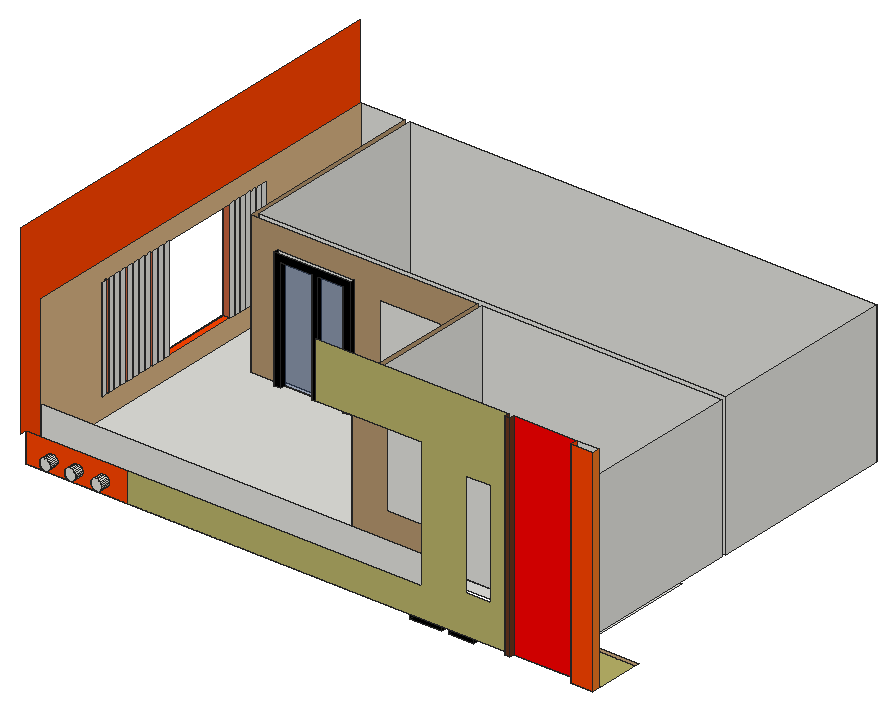
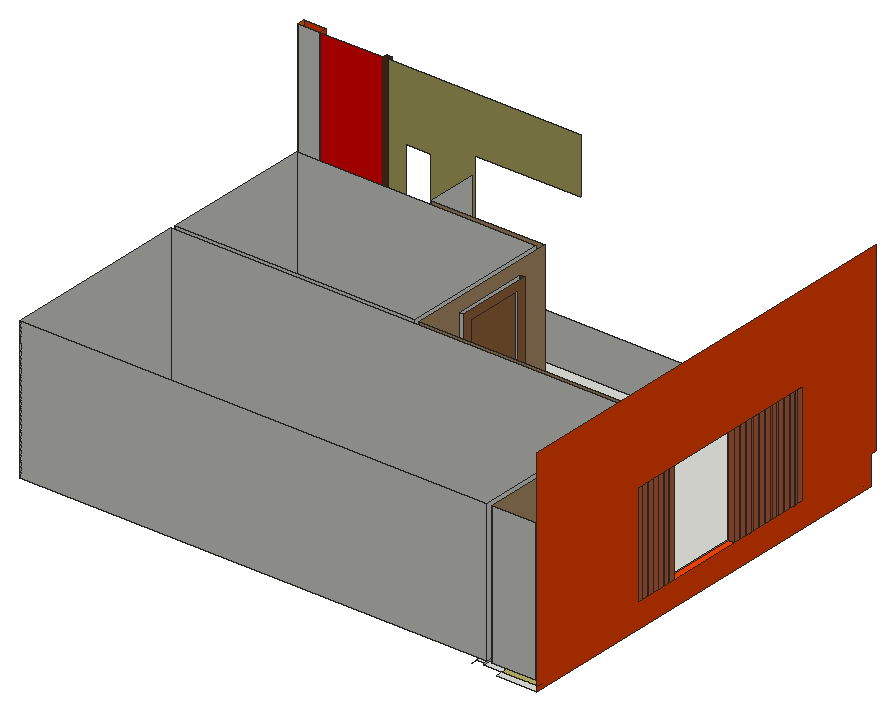
# SketchUp Ruby script. Lengths in inches.
U = 1.inch
M = Sketchup.active_model
def pt(a) = Geom::Point3d.new(a.map { |v| v * U })
def face(e, loops, mat)
  f = e.add_face(loops[0].map { |a| pt(a) })
  loops[1..].each { |l| e.add_face(l.map { |a| pt(a) }).erase! }
  f.material = f.back_material = mat if mat
  f
end
# faces: each face lists its corners as indices into pts; further lists are holes
def faces(e, pts, list, mat = nil) = list.each { |f| face(e, (f[0].is_a?(Array) ? f : [f]).map { |l| l.map { |i| pts[i] } }, mat) }
# xy, xz, yz: faces in a plane at the given z, y or x. An outline is a flat list of corners, or four numbers for a rectangle; further outlines are holes
def ring(l) = l.size == 4 ? [[l[0], l[1]], [l[2], l[1]], [l[2], l[3]], [l[0], l[3]]] : l.each_slice(2).to_a
def flat(e, list, mat, &to3) = list.each { |f| face(e, (f[0].is_a?(Array) ? f : [f]).map { |l| ring(l).map { |u, v| to3.(u, v) } }, mat) }
def xy(e, z, list, mat = nil) = flat(e, list, mat) { |x, y| [x, y, z] }
def xz(e, y, list, mat = nil) = flat(e, list, mat) { |x, z| [x, y, z] }
def yz(e, x, list, mat = nil) = flat(e, list, mat) { |y, z| [x, y, z] }
def lines(e, pts, list) = list.each { |a, b| e.add_line(pt(pts[a]), pt(pts[b])) }
# prism: a flat outline (further loops are holes) pulled along v
def prism(e, loops, v, mat = nil)
  f = face(e, loops, mat); d = Geom::Vector3d.new(v.map { |x| x * U })
  f.pushpull(f.normal.samedirection?(d) ? d.length : -d.length)
end
def box(e, o, s, mat = nil) = prism(e, [[o, [o[0] + s[0], o[1], o[2]], [o[0] + s[0], o[1] + s[1], o[2]], [o[0], o[1] + s[1], o[2]]]], [0, 0, s[2]], mat)
def at(x, y, z, deg = 0) = Geom::Transformation.translation(pt([x, y, z])) * Geom::Transformation.rotation(ORIGIN, Z_AXIS, deg.degrees)
def axes(o, x, y, z) = Geom::Transformation.new([*x, 0, *y, 0, *z, 0, *pt(o).to_a, 1])
def part(name) = M.definitions.add(name)
# library, detail: a bought-in or finely detailed component or shape, given as its bounding box
def library(name, o, s) = part(name).tap { |d| box(d.entities, o, s) }
def detail(e, o, s) = box(e.add_group.entities, o, s)
def put(e, d, t, mat = nil) = e.add_instance(d, t).tap { |i| i.material = mat if mat }
def group(e, t, mat = nil) = e.add_group.tap { |g| g.transformation = t; g.material = mat if mat }.entities
root = M.entities
M.materials.add("[0020_Red]").color = [255, 0, 0]
M.materials.add("[0024_OrangeRed]").color = [255, 69, 0]
M.materials.add("[0025_Coral]").color = [198, 99, 62]
M.materials.add("[0036_BurlyWood]").color = [181, 150, 110]
M.materials.add("[0036_BurlyWood]4").color = [216, 179, 131]
M.materials.add("[0041_Chocolate]1").color = [239, 119, 34]
M.materials.add("[0042_Sienna]").color = [104, 53, 29]
M.materials.add("[0057_DarkKhaki]").color = [186, 180, 105]
M.materials.add("[0137_Black]").color = [0, 0, 0]
M.materials.add("[Color M09]").color = [0, 0, 0]
M.materials.add("[Translucent Glass Blue]").color = [51, 76, 122]
M.materials["[Translucent Glass Blue]"].alpha = 0.5
M.materials.add("[Translucent Glass Gray]").color = [165, 165, 165]
M.materials["[Translucent Glass Gray]"].alpha = 0.5
M.materials.add("[Wood Bamboo]").color = [196, 88, 55]
M.materials.add("[Wood Floor Parquet]").color = [145, 89, 39]
M.materials.add("[Wood Floor]").color = [155, 105, 61]
xy(root,130.33,[[443.09,303.3125,483.76,309.3125],[492.14,303.3125,524.43,309.3125]],"[0137_Black]")
xy(root,132.36,[[129.72,453.875,217.79,454.875]],"[Wood Bamboo]")
xy(root,138.4375,[[379.5,353.72,382.5,429.09]],"[Wood Floor Parquet]")
xy(root,140.42,[[254.5625,454.875,298.59,457.875],[303.24,454.875,342.625,457.875]],"[0137_Black]")
xy(root,144.3,[[379.5,347.86,385.5,434.95]],"[Wood Floor Parquet]")
xy(root,144.99,[[443.09,303.3125,483.76,309.3125],[492.14,303.3125,524.43,309.3125]],"[0137_Black]")
xy(root,147.14,[[247.84,454.875,349.34,457.875]])
xy(root,153.6875,[[129.72,451.875,217.79,454.875]],"[Wood Bamboo]")
xy(root,155.1,[[432.98,303.3125,534.54,309.3125]],"[0137_Black]")
xy(root,159.6875,[[123.72,451.875,223.79,457.875]],"[Wood Bamboo]")
xy(root,177.375,[[51.5625,457.875,74.75,463.875],[51.5625,463.875,74.75,767.8125],[0,767.8125,51.5625,776.8125]])
xy(root,177.375,[[537.22,303.3125,730.1875,309.3125]],"[0036_BurlyWood]")
xy(root,177.375,[[701.81,236.125,730.1875,245.125]],"[0041_Chocolate]1")
xy(root,177.375,[[615.29,239.125,615.29,245.125,0,245.125,0,248.25,730.1875,248.25,730.1875,245.125,621.57,245.125,621.57,239.125],[0,248.25,0,767.8125,51.5625,767.8125,51.5625,457.875,385.5,457.875,385.5,309.3125,537.22,309.3125,537.22,303.3125,730.1875,303.3125,730.1875,248.25]],"[0057_DarkKhaki]")
xy(root,180,[[385.5,309.3125,391.5,315.3125],[391.5,315.3125,665.75,457.875],[74.75,457.875,83.75,463.875],[74.75,463.875,83.75,767.8125]])
xy(root,183,[[9,257.25,498.8125,257.25,498.8125,321.9375,354.4375,321.9375,354.4375,361.01,348.4375,361.01,348.4375,372.41,351.4375,372.41,351.4375,446.78,348.4375,446.78,348.4375,458.18,354.4375,458.18,354.4375,521.4375,197.41,521.4375,197.41,515.4375,188.31,515.4375,188.31,521.4375,155.35,521.4375,155.35,515.4375,148.77,515.4375,148.77,521.4375,109.24,521.4375,109.24,515.4375,100.13,515.4375,100.13,521.4375,65.25,521.4375,65.25,767.8125,9,767.8125],[360.4375,327.9375,665.75,521.4375],[348.4375,361.01,354.4375,372.41],[351.4375,372.41,354.4375,446.78],[348.4375,446.78,354.4375,458.18],
  [100.13,515.4375,109.24,521.4375],[148.77,515.4375,155.35,521.4375],[188.31,515.4375,197.41,521.4375],[71.25,527.4375,665.75,767.8125]])
xy(root,208.56,[[0,355.7,9,361.9],[0,365.65,9,365.7],[0,365.7,9,371.9],[0,375.7,9,381.9],[0,385.7,9,391.9],
  [0,395.7,9,401.9],[0,405.7,9,411.9],[0,415.7,9,421.9],[0,425.7,9,431.9],[0,435.7,9,441.9],
  [0,445.7,9,451.9],[0,455.7,9,461.9],[0,559.26,9,565.46],[0,565.46,9,567.7],[0,567.7,9,573.9],
  [0,573.9,9,576.14],[0,576.14,9,582.34],[0,582.34,9,584.57],[0,584.57,9,590.78],[0,590.78,9,593.01],
  [0,593.01,9,599.21],[0,599.21,9,601.45],[0,601.45,9,607.65],[0,607.65,9,609.89],[0,609.89,9,616.09],
  [0,616.09,9,616.14]])
xy(root,208.56,[[0,461.9,9,559.26]],"[0024_OrangeRed]")
xy(root,208.56,[[0,352.64,9,355.7],[0,361.9,9,365.65],[0,371.9,9,375.7],[0,381.9,9,385.7],[0,391.9,9,395.7],
  [0,401.9,9,405.7],[0,411.9,9,415.7],[0,421.9,9,425.7],[0,431.9,9,435.7],[0,441.9,9,445.7],
  [0,451.9,9,455.7]],"[0025_Coral]")
xz(root,233.5625,[[33.6875,185.625,35.55,185.87,37.28,186.59,38.77,187.73,39.91,189.22,40.63,190.95,40.875,192.8125,40.63,194.67,39.91,196.41,38.77,197.9,37.28,199.04,35.55,199.76,33.6875,200,31.83,199.76,30.09,199.04,28.6,197.9,27.46,196.41,26.74,194.67,26.5,192.8125,26.74,190.95,27.46,189.22,28.6,187.73,30.09,186.59,31.83,185.87],[65.6875,185.625,67.55,185.87,69.28,186.59,70.77,187.73,71.91,189.22,72.63,190.95,72.875,192.8125,72.63,194.67,71.91,196.41,70.77,197.9,69.28,199.04,67.55,199.76,65.6875,200,63.83,199.76,62.09,199.04,60.6,197.9,59.46,196.41,58.74,194.67,58.5,192.8125,58.74,190.95,59.46,189.22,60.6,187.73,62.09,186.59,63.83,185.87],[99.0625,185.625,100.92,185.87,102.66,186.59,104.14,187.73,105.29,189.22,106,190.95,106.25,192.8125,106,194.67,105.29,196.41,104.14,197.9,102.66,199.04,100.92,199.76,99.0625,200,97.2,199.76,95.47,199.04,93.98,197.9,92.84,196.41,92.12,194.67,91.875,192.8125,92.12,190.95,92.84,189.22,93.98,187.73,95.47,186.59,97.2,185.87]])
xz(root,236.125,[[701.81,177.375,730.1875,450]],"[0024_OrangeRed]")
xz(root,239.125,[[615.29,177.375,621.57,450]],"[0042_Sienna]")
xz(root,245.125,[[701.81,177.375,730.1875,450]])
xz(root,245.125,[[621.57,177.375,701.81,450]],"[0020_Red]")
xz(root,245.125,[[[0,177.375,130.26,214.625],[99.0625,185.625,97.2,185.87,95.47,186.59,93.98,187.73,92.84,189.22,92.12,190.95,91.875,192.8125,92.12,194.67,92.84,196.41,93.98,197.9,95.47,199.04,97.2,199.76,99.0625,200,100.92,199.76,102.66,199.04,104.14,197.9,105.29,196.41,106,194.67,106.25,192.8125,106,190.95,105.29,189.22,104.14,187.73,102.66,186.59,100.92,185.87],[65.6875,185.625,63.83,185.87,62.09,186.59,60.6,187.73,59.46,189.22,58.74,190.95,58.5,192.8125,58.74,194.67,59.46,196.41,60.6,197.9,62.09,199.04,63.83,199.76,65.6875,200,67.55,199.76,69.28,199.04,70.77,197.9,71.91,196.41,72.63,194.67,72.875,192.8125,72.63,190.95,71.91,189.22,70.77,187.73,69.28,186.59,67.55,185.87],[33.6875,185.625,31.83,185.87,30.09,186.59,28.6,187.73,27.46,189.22,26.74,190.95,26.5,192.8125,26.74,194.67,27.46,196.41,28.6,197.9,30.09,199.04,31.83,199.76,33.6875,200,35.55,199.76,37.28,199.04,38.77,197.9,39.91,196.41,40.63,194.67,40.875,192.8125,40.63,190.95,39.91,189.22,38.77,187.73,37.28,186.59,35.55,185.87]]],"[0024_OrangeRed]")
xz(root,245.125,[[[130.26,177.375,615.29,177.375,615.29,450,369.99,450,369.99,378.625,504.125,378.625,504.125,214.625,130.26,214.625],[561.28,226.86,593.09,360.8]]],"[0057_DarkKhaki]")
xz(root,257.25,[[9,183,498.8125,243]])
xz(root,309.3125,[[385.5,177.375,391.5,180]])
xz(root,309.3125,[[443.09,130.33,483.76,144.99],[492.14,130.33,524.43,144.99]],"[Translucent Glass Gray]")
xz(root,321.9375,[[[354.4375,183,498.8125,363],[398.32,228.95,478.64,338.07]]],"[0036_BurlyWood]")
xz(root,327.9375,[[360.4375,183,665.75,363]])
xz(root,352.64,[[0,208.56,9,339.56]],"[0025_Coral]")
xz(root,355.7,[[0,208.56,9,339.56]],"[0025_Coral]")
xz(root,361.01,[[348.4375,183,354.4375,345.77]],"[Wood Floor]")
xz(root,361.9,[[0,208.56,9,339.56]],"[0025_Coral]")
xz(root,365.65,[[0,208.56,9,339.56]],"[0025_Coral]")
xz(root,371.9,[[0,208.56,9,339.56]],"[0025_Coral]")
xz(root,372.41,[[348.4375,183,351.4375,334.375]])
xz(root,375.7,[[0,208.56,9,339.56]],"[0025_Coral]")
xz(root,381.9,[[0,208.56,9,339.56]],"[0025_Coral]")
xz(root,385.7,[[0,208.56,9,339.56]],"[0025_Coral]")
xz(root,391.9,[[0,208.56,9,339.56]],"[0025_Coral]")
xz(root,395.7,[[0,208.56,9,339.56]],"[0025_Coral]")
xz(root,401.9,[[0,208.56,9,339.56]],"[0025_Coral]")
xz(root,405.7,[[0,208.56,9,339.56]],"[0025_Coral]")
xz(root,411.9,[[0,208.56,9,339.56]],"[0025_Coral]")
xz(root,415.7,[[0,208.56,9,339.56]],"[0025_Coral]")
xz(root,421.9,[[0,208.56,9,339.56]],"[0025_Coral]")
xz(root,425.7,[[0,208.56,9,339.56]],"[0025_Coral]")
xz(root,431.9,[[0,208.56,9,339.56]],"[0025_Coral]")
xz(root,435.7,[[0,208.56,9,339.56]],"[0025_Coral]")
xz(root,441.9,[[0,208.56,9,339.56]],"[0025_Coral]")
xz(root,445.7,[[0,208.56,9,339.56]],"[0025_Coral]")
xz(root,446.78,[[348.4375,183,351.4375,334.375]],"[Wood Floor]")
xz(root,451.9,[[0,208.56,9,339.56]],"[0025_Coral]")
xz(root,454.875,[[129.72,132.36,217.79,153.6875]],"[Wood Bamboo]")
xz(root,455.7,[[0,208.56,9,339.69]],"[0025_Coral]")
xz(root,457.875,[[74.75,177.375,83.75,180]])
xz(root,458.18,[[348.4375,183,354.4375,345.77]])
xz(root,461.9,[[0,208.56,9,339.69]],"[0025_Coral]")
xz(root,515.4375,[[100.13,183,109.24,183,109.24,326.0625,148.77,326.0625,148.77,183,155.35,183,155.35,326.0625,188.31,326.0625,188.31,183,197.41,183,197.41,335.17,100.13,335.17]],"[0137_Black]")
xz(root,521.4375,[[100.13,173.89,197.41,183],[360.4375,183,665.75,363]])
xz(root,521.4375,[[[65.25,183,100.13,183,100.13,335.17,197.41,335.17,197.41,183,354.4375,183,354.4375,363,65.25,363],[230.26,235.22,307.58,323.78]]],"[0036_BurlyWood]")
xz(root,521.4375,[[109.24,183,148.77,326.0625],[155.35,183,188.31,326.0625]],"[Translucent Glass Blue]")
xz(root,527.4375,[[71.25,183,665.75,363]])
xz(root,559.26,[[0,208.56,9,339.56]],"[0025_Coral]")
xz(root,565.46,[[0,208.56,9,339.56]],"[0025_Coral]")
xz(root,567.7,[[0,208.56,9,339.56]],"[0025_Coral]")
xz(root,573.9,[[0,208.56,9,339.56]],"[0025_Coral]")
xz(root,576.14,[[0,208.56,9,339.56]],"[0025_Coral]")
xz(root,582.34,[[0,208.56,9,339.56]],"[0025_Coral]")
xz(root,584.57,[[0,208.56,9,339.56]],"[0025_Coral]")
xz(root,590.78,[[0,208.56,9,339.56]],"[0025_Coral]")
xz(root,593.01,[[0,208.56,9,339.56]],"[0025_Coral]")
xz(root,599.21,[[0,208.56,9,339.56]],"[0025_Coral]")
xz(root,601.45,[[0,208.56,9,339.56]],"[0025_Coral]")
xz(root,607.65,[[0,208.56,9,339.56]],"[0025_Coral]")
xz(root,609.89,[[0,208.56,9,339.56]],"[0025_Coral]")
xz(root,616.09,[[0,208.56,9,339.56]])
xz(root,616.14,[[0,208.56,9,339.56]])
xz(root,767.8125,[[9,183,65.25,363],[71.25,183,665.75,363]])
yz(root,0,[[365.65,208.56,365.7,339.56]])
yz(root,0,[[[245.125,177.375,245.125,214.625,236.25,214.625,236.25,450,776.8125,450,776.8125,177.375],[352.64,208.56,616.14,339.56]]],"[0024_OrangeRed]")
yz(root,0,[[355.7,208.56,361.9,339.56],[365.7,208.56,371.9,339.56],[375.7,208.56,381.9,339.56],[385.7,208.56,391.9,339.56],[395.7,208.56,401.9,339.56],
  [405.7,208.56,411.9,339.56],[415.7,208.56,421.9,339.56],[425.7,208.56,431.9,339.56],[435.7,208.56,441.9,339.56],[445.7,208.56,451.9,339.56],
  [455.7,208.56,461.9,339.56],[559.26,208.56,565.46,339.56],[567.7,208.56,573.9,339.56],[576.14,208.56,582.34,339.56],[584.57,208.56,590.78,339.56],
  [593.01,208.56,599.21,339.56],[601.45,208.56,607.65,339.56],[609.89,208.56,616.09,339.56]],"[0025_Coral]")
yz(root,9,[[355.7,208.56,361.9,339.56],[365.65,208.56,365.7,339.56],[365.7,208.56,371.9,339.56],[375.7,208.56,381.9,339.56],[385.7,208.56,391.9,339.56],
  [395.7,208.56,401.9,339.56],[405.7,208.56,411.9,339.56],[415.7,208.56,421.9,339.56],[425.7,208.56,431.9,339.56],[435.7,208.56,441.9,339.56],
  [445.7,208.56,451.9,339.56],[455.7,208.56,461.9,339.56],[559.26,208.56,565.46,339.56],[567.7,208.56,573.9,339.56],[576.14,208.56,582.34,339.56],
  [584.57,208.56,590.78,339.56],[593.01,208.56,599.21,339.56],[601.45,208.56,607.65,339.56],[609.89,208.56,616.09,339.56]])
yz(root,9,[[[257.25,183,767.8125,363],[352.64,208.56,616.14,339.56]]],"[0036_BurlyWood]4")
yz(root,65.25,[[521.4375,183,767.8125,363]],"[0036_BurlyWood]")
yz(root,71.25,[[527.4375,183,767.8125,363]])
yz(root,74.75,[[457.875,177.375,463.875,180],[463.875,177.375,767.8125,180]])
yz(root,100.13,[[515.4375,183,521.4375,335.17]],"[Color M09]")
yz(root,109.24,[[515.4375,183,521.4375,326.0625]],"[0137_Black]")
yz(root,148.77,[[515.4375,183,521.4375,326.0625]],"[0137_Black]")
yz(root,155.35,[[515.4375,183,521.4375,326.0625]],"[0137_Black]")
yz(root,188.31,[[515.4375,183,521.4375,326.0625]],"[0137_Black]")
yz(root,197.41,[[515.4375,183,521.4375,335.17]],"[0137_Black]")
yz(root,348.4375,[[361.01,183,361.01,345.77,458.18,345.77,458.18,183,446.78,183,446.78,334.375,372.41,334.375,372.41,183]],"[Wood Floor]")
yz(root,351.4375,[[[372.41,183,446.78,334.375],[427.62,258.41,430.86,259,433.84,260.41,436.36,262.55,438.23,265.26,439.34,268.36,439.61,271.65,439.02,274.89,437.6,277.87,435.47,280.38,432.76,282.25,429.66,283.36,426.37,283.63,423.13,283.04,420.15,281.63,417.64,279.49,415.76,276.78,414.66,273.68,414.39,270.4,414.98,267.15,416.39,264.17,418.52,261.66,421.23,259.79,424.34,258.68]]],"[Wood Floor]")
yz(root,354.4375,[[321.9375,183,321.9375,363,521.4375,363,521.4375,183,458.18,183,458.18,345.77,361.01,345.77,361.01,183]],"[0036_BurlyWood]")
yz(root,360.4375,[[327.9375,183,521.4375,363]])
yz(root,385.5,[[309.3125,177.375,315.3125,180]])
yz(root,443.09,[[303.3125,130.33,309.3125,144.99]],"[0137_Black]")
yz(root,483.76,[[303.3125,130.33,309.3125,144.99]],"[0137_Black]")
yz(root,492.14,[[303.3125,130.33,309.3125,144.99]],"[0137_Black]")
yz(root,498.8125,[[257.25,183,321.9375,363]])
yz(root,524.43,[[303.3125,130.33,309.3125,144.99]],"[0137_Black]")
yz(root,615.29,[[239.125,177.375,245.125,450]],"[0042_Sienna]")
yz(root,621.57,[[239.125,177.375,245.125,450]],"[0042_Sienna]")
yz(root,665.75,[[327.9375,183,521.4375,363],[527.4375,183,767.8125,363]])
yz(root,701.81,[[236.125,177.375,245.125,450]],"[0024_OrangeRed]")
yz(root,730.1875,[[236.125,177.375,245.125,450]],"[0041_Chocolate]1")
p = [[31.83,245.125,185.87],[33.6875,245.125,185.625],[33.6875,233.5625,185.625],[31.83,233.5625,185.87],[35.55,245.125,185.87],[35.55,233.5625,185.87],
  [63.83,245.125,185.87],[65.6875,245.125,185.625],[65.6875,233.5625,185.625],[63.83,233.5625,185.87],[67.55,245.125,185.87],[67.55,233.5625,185.87],
  [97.2,245.125,185.87],[99.0625,245.125,185.625],[99.0625,233.5625,185.625],[97.2,233.5625,185.87],[100.92,245.125,185.87],[100.92,233.5625,185.87],
  [30.09,245.125,186.59],[30.09,233.5625,186.59],[37.28,245.125,186.59],[37.28,233.5625,186.59],[62.09,245.125,186.59],[62.09,233.5625,186.59],
  [69.28,245.125,186.59],[69.28,233.5625,186.59],[95.47,245.125,186.59],[95.47,233.5625,186.59],[102.66,245.125,186.59],[102.66,233.5625,186.59],
  [28.6,245.125,187.73],[28.6,233.5625,187.73],[38.77,245.125,187.73],[38.77,233.5625,187.73],[60.6,245.125,187.73],[60.6,233.5625,187.73],
  [70.77,245.125,187.73],[70.77,233.5625,187.73],[93.98,245.125,187.73],[93.98,233.5625,187.73],[104.14,245.125,187.73],[104.14,233.5625,187.73],
  [27.46,245.125,189.22],[27.46,233.5625,189.22],[39.91,245.125,189.22],[39.91,233.5625,189.22],[59.46,245.125,189.22],[59.46,233.5625,189.22],
  [71.91,245.125,189.22],[71.91,233.5625,189.22],[92.84,245.125,189.22],[92.84,233.5625,189.22],[105.29,245.125,189.22],[105.29,233.5625,189.22],
  [26.74,245.125,190.95],[26.74,233.5625,190.95],[40.63,245.125,190.95],[40.63,233.5625,190.95],[58.74,245.125,190.95],[58.74,233.5625,190.95],
  [72.63,245.125,190.95],[72.63,233.5625,190.95],[92.12,245.125,190.95],[92.12,233.5625,190.95],[106,245.125,190.95],[106,233.5625,190.95],
  [26.5,245.125,192.8125],[26.5,233.5625,192.8125],[40.875,245.125,192.8125],[40.875,233.5625,192.8125],[58.5,245.125,192.8125],[58.5,233.5625,192.8125],
  [72.875,245.125,192.8125],[72.875,233.5625,192.8125],[91.875,245.125,192.8125],[91.875,233.5625,192.8125],[106.25,245.125,192.8125],[106.25,233.5625,192.8125],
  [26.74,245.125,194.67],[26.74,233.5625,194.67],[40.63,245.125,194.67],[40.63,233.5625,194.67],[58.74,245.125,194.67],[58.74,233.5625,194.67],
  [72.63,245.125,194.67],[72.63,233.5625,194.67],[92.12,245.125,194.67],[92.12,233.5625,194.67],[106,245.125,194.67],[106,233.5625,194.67],
  [27.46,245.125,196.41],[27.46,233.5625,196.41],[39.91,245.125,196.41],[39.91,233.5625,196.41],[59.46,245.125,196.41],[59.46,233.5625,196.41],
  [71.91,245.125,196.41],[71.91,233.5625,196.41],[92.84,245.125,196.41],[92.84,233.5625,196.41],[105.29,245.125,196.41],[105.29,233.5625,196.41],
  [28.6,245.125,197.9],[28.6,233.5625,197.9],[38.77,245.125,197.9],[38.77,233.5625,197.9],[60.6,245.125,197.9],[60.6,233.5625,197.9],
  [70.77,245.125,197.9],[70.77,233.5625,197.9],[93.98,245.125,197.9],[93.98,233.5625,197.9],[104.14,245.125,197.9],[104.14,233.5625,197.9],
  [30.09,245.125,199.04],[30.09,233.5625,199.04],[37.28,245.125,199.04],[37.28,233.5625,199.04],[62.09,245.125,199.04],[62.09,233.5625,199.04],
  [69.28,245.125,199.04],[69.28,233.5625,199.04],[95.47,245.125,199.04],[95.47,233.5625,199.04],[102.66,245.125,199.04],[102.66,233.5625,199.04],
  [31.83,245.125,199.76],[31.83,233.5625,199.76],[35.55,245.125,199.76],[35.55,233.5625,199.76],[63.83,245.125,199.76],[63.83,233.5625,199.76],
  [67.55,245.125,199.76],[67.55,233.5625,199.76],[97.2,245.125,199.76],[97.2,233.5625,199.76],[100.92,245.125,199.76],[100.92,233.5625,199.76],
  [33.6875,245.125,200],[33.6875,233.5625,200],[65.6875,245.125,200],[65.6875,233.5625,200],[99.0625,245.125,200],[99.0625,233.5625,200],
  [83.75,767.8125,180],[83.75,767.8125,183],[83.75,776.8125,180],[0,776.8125,183],[0,767.8125,183],[354.4375,458.18,183],
  [354.4375,458.18,171.6],[9,257.25,183],[0,257.25,183],[9,767.8125,183]]
faces(root,p,[[0,1,2,3],[1,4,5,2],[6,7,8,9],[7,10,11,8],[12,13,14,15],[13,16,17,14],[18,0,3,19],[4,20,21,5],
  [22,6,9,23],[10,24,25,11],[26,12,15,27],[16,28,29,17],[30,18,19,31],[20,32,33,21],[34,22,23,35],[24,36,37,25],
  [38,26,27,39],[28,40,41,29],[42,30,31,43],[32,44,45,33],[46,34,35,47],[36,48,49,37],[50,38,39,51],[40,52,53,41],
  [54,42,43,55],[44,56,57,45],[58,46,47,59],[48,60,61,49],[62,50,51,63],[52,64,65,53],[66,54,55,67],[56,68,69,57],
  [70,58,59,71],[60,72,73,61],[74,62,63,75],[64,76,77,65],[78,66,67,79],[68,80,81,69],[82,70,71,83],[72,84,85,73],
  [86,74,75,87],[76,88,89,77],[90,78,79,91],[80,92,93,81],[94,82,83,95],[84,96,97,85],[98,86,87,99],[88,100,101,89],
  [102,90,91,103],[92,104,105,93],[106,94,95,107],[96,108,109,97],[110,98,99,111],[100,112,113,101],[114,102,103,115],[104,116,117,105],
  [118,106,107,119],[108,120,121,109],[122,110,111,123],[112,124,125,113],[126,114,115,127],[116,128,129,117],[130,118,119,131],[120,132,133,121],
  [134,122,123,135],[124,136,137,125],[138,126,127,139],[128,138,139,129],[140,130,131,141],[132,140,141,133],[142,134,135,143],[136,142,143,137]])
lines(root,p,[[144,145],[144,146],[147,148],[149,150],[151,152],[153,148]])
